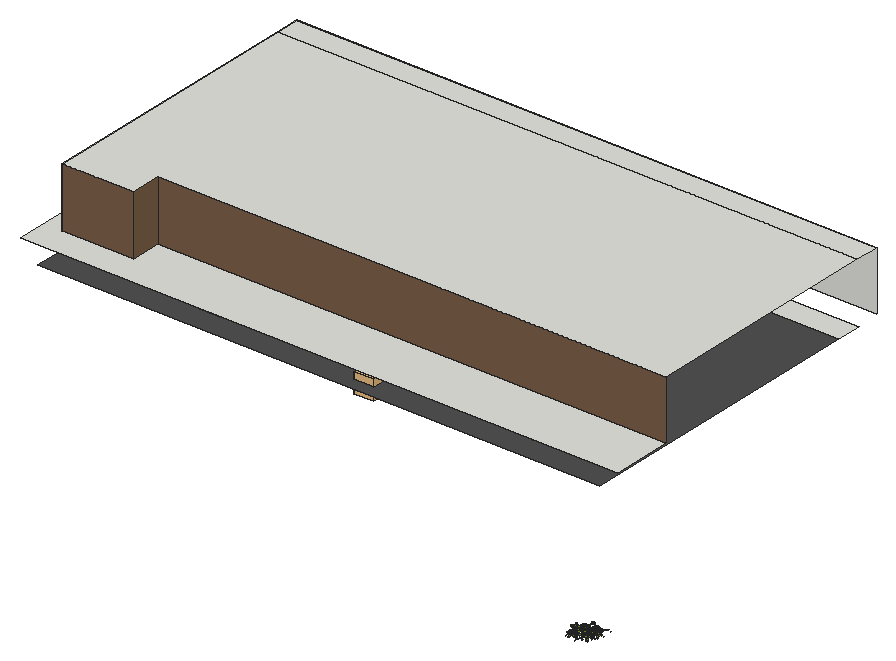
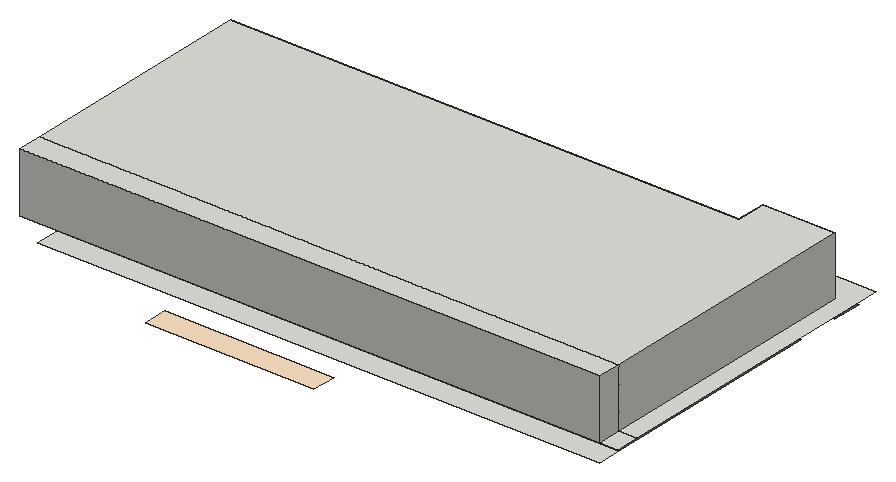
# SketchUp Ruby script. Lengths in inches.
U = 1.inch
M = Sketchup.active_model
def pt(a) = Geom::Point3d.new(a.map { |v| v * U })
def face(e, loops, mat)
  f = e.add_face(loops[0].map { |a| pt(a) })
  loops[1..].each { |l| e.add_face(l.map { |a| pt(a) }).erase! }
  f.material = f.back_material = mat if mat
  f
end
# faces: each face lists its corners as indices into pts; further lists are holes
def faces(e, pts, list, mat = nil) = list.each { |f| face(e, (f[0].is_a?(Array) ? f : [f]).map { |l| l.map { |i| pts[i] } }, mat) }
# xy, xz, yz: faces in a plane at the given z, y or x. An outline is a flat list of corners, or four numbers for a rectangle; further outlines are holes
def ring(l) = l.size == 4 ? [[l[0], l[1]], [l[2], l[1]], [l[2], l[3]], [l[0], l[3]]] : l.each_slice(2).to_a
def flat(e, list, mat, &to3) = list.each { |f| face(e, (f[0].is_a?(Array) ? f : [f]).map { |l| ring(l).map { |u, v| to3.(u, v) } }, mat) }
def xy(e, z, list, mat = nil) = flat(e, list, mat) { |x, y| [x, y, z] }
def xz(e, y, list, mat = nil) = flat(e, list, mat) { |x, z| [x, y, z] }
def yz(e, x, list, mat = nil) = flat(e, list, mat) { |y, z| [x, y, z] }
def lines(e, pts, list) = list.each { |a, b| e.add_line(pt(pts[a]), pt(pts[b])) }
# prism: a flat outline (further loops are holes) pulled along v
def prism(e, loops, v, mat = nil)
  f = face(e, loops, mat); d = Geom::Vector3d.new(v.map { |x| x * U })
  f.pushpull(f.normal.samedirection?(d) ? d.length : -d.length)
end
def box(e, o, s, mat = nil) = prism(e, [[o, [o[0] + s[0], o[1], o[2]], [o[0] + s[0], o[1] + s[1], o[2]], [o[0], o[1] + s[1], o[2]]]], [0, 0, s[2]], mat)
def at(x, y, z, deg = 0) = Geom::Transformation.translation(pt([x, y, z])) * Geom::Transformation.rotation(ORIGIN, Z_AXIS, deg.degrees)
def axes(o, x, y, z) = Geom::Transformation.new([*x, 0, *y, 0, *z, 0, *pt(o).to_a, 1])
def part(name) = M.definitions.add(name)
# library, detail: a bought-in or finely detailed component or shape, given as its bounding box
def library(name, o, s) = part(name).tap { |d| box(d.entities, o, s) }
def detail(e, o, s) = box(e.add_group.entities, o, s)
def put(e, d, t, mat = nil) = e.add_instance(d, t).tap { |i| i.material = mat if mat }
def group(e, t, mat = nil) = e.add_group.tap { |g| g.transformation = t; g.material = mat if mat }.entities
root = M.entities
M.materials.add("[0012_Bisque]").color = [255, 228, 196]
M.materials.add("[0050_LemonChiffon]").color = [255, 250, 205]
M.materials.add("[0054_LightYellow]").color = [255, 255, 224]
M.materials.add("[0061_OliveDrab]").color = [107, 142, 35]
M.materials.add("[0135_DarkGray]").color = [81, 81, 81]
M.materials.add("[Cladding Siding Tan]").color = [124, 97, 73]
c1 = library("Sphere Light\#1",[-9.875,-9.875,-9.875],[19.75,19.75,19.75])
c2 = library("Sphere Light\#2",[-9.875,-9.875,-9.875],[19.75,19.75,19.75])
c3 = library("Sphere Light",[-9.875,-9.875,-9.875],[19.75,19.75,19.75])
xy(root,667.5,[[304.95,312,474.45,336]],"[0012_Bisque]")
xy(root,702,[[18,312,582,336]])
xy(root,702,[[170.5,36.91,167.95,37.24,165.5625,38.23,163.52,39.8,161.95,41.85,160.96,44.23,160.625,46.78,160.96,49.34,161.95,51.72,163.52,53.77,165.5625,55.34,167.95,56.32,170.5,56.66,173.06,56.32,175.4375,55.34,177.48,53.77,179.05,51.72,180.04,49.34,180.375,46.78,180.04,44.23,179.05,41.85,177.48,39.8,175.4375,38.23,173.06,37.24]],"[0050_LemonChiffon]")
xy(root,702,[[335.0625,36.91,332.51,37.24,330.125,38.23,328.08,39.8,326.51,41.85,325.52,44.23,325.1875,46.78,325.52,49.34,326.51,51.72,328.08,53.77,330.125,55.34,332.51,56.32,335.0625,56.66,337.62,56.32,340,55.34,342.05,53.77,343.62,51.72,344.6,49.34,344.9375,46.78,344.6,44.23,343.62,41.85,342.05,39.8,340,38.23,337.62,37.24],[504.5625,36.91,502.01,37.24,499.625,38.23,497.58,39.8,496.01,41.85,495.02,44.23,494.6875,46.78,495.02,49.34,496.01,51.72,497.58,53.77,499.625,55.34,502.01,56.32,504.5625,56.66,507.12,56.32,509.5,55.34,511.55,53.77,513.12,51.72,514.1,49.34,514.4375,46.78,514.1,44.23,513.12,41.85,511.55,39.8,509.5,38.23,507.12,37.24]],"[0054_LightYellow]")
xy(root,702,[[[18,12,18,42,90,42,90,72,240,72,240,84,18,84,18,312,582,312,582,12],[170.5,36.91,173.06,37.24,175.4375,38.23,177.48,39.8,179.05,41.85,180.04,44.23,180.375,46.78,180.04,49.34,179.05,51.72,177.48,53.77,175.4375,55.34,173.06,56.32,170.5,56.66,167.95,56.32,165.5625,55.34,163.52,53.77,161.95,51.72,160.96,49.34,160.625,46.78,160.96,44.23,161.95,41.85,163.52,39.8,165.5625,38.23,167.95,37.24],[335.0625,36.91,337.62,37.24,340,38.23,342.05,39.8,343.62,41.85,344.6,44.23,344.9375,46.78,344.6,49.34,343.62,51.72,342.05,53.77,340,55.34,337.62,56.32,335.0625,56.66,332.51,56.32,330.125,55.34,328.08,53.77,326.51,51.72,325.52,49.34,325.1875,46.78,325.52,44.23,326.51,41.85,328.08,39.8,330.125,38.23,332.51,37.24],[504.5625,36.91,507.12,37.24,509.5,38.23,511.55,39.8,513.12,41.85,514.1,44.23,514.4375,46.78,514.1,49.34,513.12,51.72,511.55,53.77,509.5,55.34,507.12,56.32,504.5625,56.66,502.01,56.32,499.625,55.34,497.58,53.77,496.01,51.72,495.02,49.34,494.6875,46.78,495.02,44.23,496.01,41.85,497.58,39.8,499.625,38.23,502.01,37.24]]],"[0135_DarkGray]")
xy(root,720,[[0,12,600,12,600,72,90,72,90,42,18,42,18,312,0,312],[0,312,18,336]])
xy(root,780,[[18,42,90,42,90,72,600,72,600,312,18,312],[18,312,600,336]])
xz(root,42,[[18,720,90,780]],"[Cladding Siding Tan]")
xz(root,72,[[90,720,600,780]],"[Cladding Siding Tan]")
xz(root,336,[[18,720,600,780]])
yz(root,18,[[42,720,312,780],[312,720,336,780]])
yz(root,90,[[42,720,72,780]],"[Cladding Siding Tan]")
p = [[564.29,5.1875,560.78],[564.12,5.33,560.78],[562.93,3.75,559.05],[561.79,8.16,559.04],[561.59,8.49,559.04],[560.2,7.625,561.09],
  [560.36,7.35,561.09],[573.22,17.34,559.04],[573.47,17.11,559.04],[574.44,18.17,561.23],[574.25,18.36,561.23],[559.27,9.62,561],
  [559.09,9.66,561],[558.8,7.87,559.1],[566.09,10.13,560.93],[565.87,10.1,560.93],[566.23,8.25,559.11],[554.1,19.08,560.81],
  [554.27,19.22,560.81],[552.92,20.64,559.06],[549.52,22.11,560.79],[549.58,22.3125,560.79],[547.63,22.78,559.09],[567.24,8.58,559.22],
  [566.95,8.82,559.22],[565.76,7.36,561.05],[566,7.16,561.05],[570.125,9.75,559.22],[569.9,9.45,559.22],[570.88,8.76,561.55],
  [571.0625,9.01,561.55],[556.11,23.33,561.13],[555.97,23.45,561.13],[554.89,22.05,559.1875],[571.21,27.76,559.17],[571.48,27.51,559.17],
  [572.73,28.93,560.99],[572.51,29.13,560.99],[557.76,29.01,559.24],[557.83,28.63,559.24],[559.08,28.89,561.53],[559.03,29.2,561.53],
  [559.84,9.14,559.32],[559.55,9.32,559.32],[558.6875,7.88,561.34],[558.92,7.74,561.34],[557.04,9.63,559.34],[556.76,9.86,559.34],
  [555.7,8.53,561.34],[555.93,8.34,561.34],[559.59,9.21,559.33],[559.21,9.31,559.33],[559.125,8.81,561.9],[559.43,8.74,561.9],
  [559.85,9.31,559.35],[560.18,9.4,559.35],[559.76,10.89,561.46],[559.48,10.82,561.46],[569.45,10.46,559.34],[569.75,10.28,559.34],
  [570.17,11.08,561.81],[569.93,11.22,561.81],[572.375,13.1875,559.3],[572.11,13.4,559.3],[571.79,12.94,561.86],[572.01,12.77,561.86],
  [553.34,16.17,559.34],[553.05,15.98,559.34],[553.48,15.37,561.85],[553.72,15.52,561.85],[557.53,17.27,561.0625],[557.37,17.39,561.0625],
  [556.28,15.83,559.26],[572.23,16.52,559.35],[572.37,16.18,559.35],[572.5,16.27,561.97],[572.39,16.54,561.97],[574.33,18.23,561.04],
  [574.2,18.04,561.04],[575.89,17.03,559.29],[550.33,19.14,560.92],[550.49,19.27,560.92],[549.12,20.79,559.27],[552.93,20.14,559.31],
  [553.14,20.4,559.31],[552,21.29,561.49],[551.82,21.08,561.49],[553.2,21.02,559.32],[552.94,21.24,559.32],[552.26,20.38,561.7],
  [552.47,20.2,561.7],[573.49,22.4,561],[573.5625,22.19,561],[575.375,22.93,559.25],[572.35,24.65,559.26],[572.42,25.02,559.26],
  [572.06,25.05,561.86],[572,24.75,561.86],[571.86,25.09,559.32],[571.74,25.43,559.32],[571.25,25.22,561.89],[571.35,24.95,561.89],
  [560.84,25.625,561.04],[561.05,25.72,561.04],[560.1,27.49,559.34],[563.4,28.35,559.34],[563.71,28.59,559.34],[563.04,29.37,561.76],
  [562.79,29.17,561.76],[569.4375,29.21,560.97],[569.57,29.07,560.97],[570.95,30.55,559.29],[555.47,10.89,559.35],[555.15,10.82,559.35],
  [555.51,9.39,561.52],[555.77,9.44,561.52],[569.34,11.16,559.43],[569.52,10.83,559.43],[570.57,11.45,561.76],[570.43,11.72,561.76],
  [554.07,13.21,559.4375],[554.42,13.3,559.4375],[554.05,14.52,561.73],[553.77,14.44,561.73],[553.33,14.41,559.36],[553.51,14.7,559.36],
  [552.36,15.38,561.62],[552.21,15.14,561.62],[553.15,15.55,559.36],[553.4375,15.78,559.36],[552.18,17.27,561.11],[551.95,17.08,561.11],
  [570.58,22.38,560.95],[570.46,22.21,560.95],[572.24,21.06,559.4],[553.25,21.39,559.39],[553.62,21.33,559.39],[553.85,23.12,561.29],
  [553.55,23.17,561.29],[558.83,28,559.41],[559.1875,28.09,559.41],[558.78,29.74,561.41],[558.49,29.67,561.41],[574.3125,31.04,560.96],
  [574.47,30.89,560.96],[575.84,32.54,559.4375],[554.22,6.35,561.21],[554.0625,6.49,561.21],[552.86,4.88,559.51],[559.92,10.61,559.5],
  [560.09,10.89,559.5],[558.37,11.94,561.17],[558.23,11.72,561.17],[568.48,11.27,559.5],[568.37,11.64,559.5],[567.33,11.29,561.89],
  [567.42,10.99,561.89],[556.67,11.94,559.5],[556.45,12.19,559.5],[555.53,11.35,561.81],[555.71,11.14,561.81],[555.46,12.43,559.49],
  [555.11,12.39,559.49],[555.25,11.41,561.93],[555.54,11.44,561.93],[561.33,11.84,559.5],[561.36,12.23,559.5],[560.08,12.3,561.79],
  [560.06,11.98,561.79],[565.09,12.41,559.5],[565.22,12.04,559.5],[566.55,12.54,561.71],[566.44,12.85,561.71],[560.24,13.86,559.5],
  [559.93,13.93,559.5],[559.59,12.2,561.45],[559.85,12.14,561.45],[565.57,14.58,559.5],[565.19,14.53,559.5],[565.48,12.67,561.33],
  [565.78,12.71,561.33],[568.1875,12.74,559.5],[568.52,12.67,559.5],[568.82,14.23,561.59],[568.55,14.29,561.59],[563.4,13.59,559.5],
  [563.23,13.25,559.5],[564,12.91,561.99],[564.14,13.1875,561.99],[558.86,13.37,561.3],[559.06,13.42,561.3],[558.46,15.28,559.54],
  [554.43,13.97,559.5],[554.75,13.8,559.5],[555.3,14.92,561.8125],[555.04,15.05,561.8125],[567.01,15.08,559.5],[566.73,14.89,559.5],
  [567.44,13.9,561.82],[567.67,14.06,561.82],[556.66,15.29,559.5],[556.42,15.56,559.5],[555.2,14.37,561.5],[555.4,14.15,561.5],
  [563.9375,14.78,559.5],[563.6875,14.99,559.5],[563.26,14.45,562.03],[563.46,14.27,562.03],[565.76,15.46,559.5],[565.6875,15.15,559.5],
  [566.84,14.92,561.85],[566.89,15.17,561.85],[561.3,15.32,559.5],[561.48,15,559.5],[562.44,15.57,561.875],[562.29,15.84,561.875],
  [557.04,15.51,559.5],[557.33,15.75,559.5],[555.99,17.27,561.17],[555.75,17.07,561.17],[562.11,18.08,559.5],[561.77,18,559.5],
  [562.26,16.15,561.3],[562.53,16.22,561.3],[564.8,16.47,559.5],[564.95,16.11,559.5],[565.97,16.61,561.87],[565.84,16.9,561.87],
  [563.02,16.39,559.5],[563.24,16.64,559.5],[561.9375,17.76,561.49],[561.76,17.55,561.49],[567.9,18.09,559.5],[567.54,18.08,559.5],
  [567.61,16.95,561.87],[567.9,16.96,561.87],[561.3,18.26,559.5],[560.99,18.06,559.5],[561.4,17.51,562.04],[561.65,17.68,562.04],
  [560.57,17.86,559.5],[560.51,18.21,559.5],[559.22,17.93,561.77],[559.28,17.65,561.77],[570.41,18.94,559.5],[570.08,18.9,559.5],
  [570.24,18.01,561.97],[570.51,18.05,561.97],[560.66,18.375,559.5],[560.93,18.1875,559.5],[561.875,19.61,561.5],[561.66,19.76,561.5],
  [563.25,19.7,559.5],[562.95,19.9,559.5],[562.25,18.8125,561.78],[562.49,18.65,561.78],[568.65,19.21,559.5],[568.49,19.48,559.5],
  [567.62,18.91,561.91],[567.76,18.69,561.91],[556.41,19.01,559.5],[556.73,18.89,559.5],[557.18,20.17,561.75],[556.92,20.27,561.75],
  [562.67,19.18,559.5],[563,19.27,559.5],[562.6,20.65,561.7],[562.34,20.58,561.7],[560.3,20.71,559.5],[560.03,20.92,559.5],
  [558.9375,19.47,561.4],[559.16,19.3,561.4],[570.66,20.8125,559.5],[570.4375,20.49,559.5],[572.02,19.46,561.33],[572.2,19.73,561.33],
  [566.75,20.12,559.5],[567.07,20.33,559.5],[566.49,21.15,561.93],[566.22,20.98,561.93],[569.2,21,559.5],[569.32,20.64,559.5],
  [571.11,21.3,561.31],[571.01,21.59,561.31],[553.97,20.71,559.5],[554.07,21.05,559.5],[552.08,21.61,561.12],[552,21.33,561.12],
  [566.52,20.66,559.5],[566.9,20.76,559.5],[566.43,22.39,561.5],[566.125,22.31,561.5],[558.6,22.79,559.5],[558.22,22.68,559.5],
  [558.7,21.09,561.53],[559.01,21.17,561.53],[558.51,21.09,559.5],[558.83,21.08,559.5],[558.84,21.78,562.03],[558.58,21.79,562.03],
  [561.125,21.4375,559.5],[561.39,21.15,559.5],[562.82,22.51,561.23],[562.6,22.75,561.23],[559.14,21.95,559.5],[558.96,21.67,559.5],
  [559.66,21.27,562],[559.8,21.5,562],[565.32,23.03,559.5],[565,23.17,559.5],[564.34,21.56,561.47],[564.6,21.45,561.47],
  [562.68,21.48,559.5],[563.04,21.65,559.5],[562.19,23.375,561.29],[561.9,23.24,561.29],[565.33,22.04,559.5],[565.26,22.37,559.5],
  [563.49,21.98,561.4],[563.55,21.71,561.4],[561.8,22.32,559.5],[561.61,22.6,559.5],[560.88,22.05,561.96],[561.04,21.82,561.96],
  [559.53,21.875,559.5],[559.84,22.04,559.5],[559.3,23,561.88],[559.05,22.87,561.88],[554.89,22.22,559.5],[555.25,22.23,559.5],
  [555.15,24.0625,561.38],[554.86,24.05,561.38],[565.91,22.61,559.5],[565.98,22.28,559.5],[566.875,22.52,561.96],[566.8125,22.78,561.96],
  [558.59,23.02,559.5],[558.43,23.3,559.5],[557.4375,22.69,561.85],[557.56,22.47,561.85],[565.38,23.52,559.5],[565.2,23.21,559.5],
  [566.52,22.48,561.65],[566.67,22.73,561.65],[569.3,23.05,559.5],[569.58,23.25,559.5],[568.69,24.39,561.69],[568.47,24.22,561.69],
  [563.03,24.21,559.5],[562.84,24.47,559.5],[561.56,23.47,561.5625],[561.71,23.26,561.5625],[566.83,25.18,559.5],[566.62,24.89,559.5],
  [568.31,23.71,561.12],[568.48,23.95,561.12],[560.31,24.77,559.5],[560.04,24.98,559.5],[559.31,23.97,561.81],[559.52,23.8,561.81],
  [564.5625,24.49,561.07],[564.71,24.32,561.07],[566.17,25.8125,559.47],[562.52,26.07,559.5],[562.29,25.76,559.5],[563.58,24.85,561.6],
  [563.76,25.1,561.6],[555.8125,26.02,559.5],[555.64,25.73,559.5],[557.01,24.97,561.61],[557.15,25.21,561.61],[558.875,26.46,559.5],
  [558.63,26.67,559.5],[557.62,25.44,561.59],[557.82,25.27,561.59],[566.09,26.05,559.5],[566.32,25.82,559.5],[567.72,27.22,561.22],
  [567.53,27.41,561.22],[565.77,27.27,559.5],[565.53,27.54,559.5],[564.14,26.22,561.3],[564.34,26.01,561.3],[563.12,13.66,561.1875],
  [562.92,13.61,561.1875],[563.52,11.61,559.6],[556.03,13.15,561.07],[556.13,13.3125,561.07],[554.27,14.375,559.56],[560.97,21.23,561.24],
  [560.93,21.41,561.24],[558.97,20.92,559.5625],[565.83,23.49,561.42],[565.7,23.3125,561.42],[567.32,22.24,559.66],[562.375,24.27,561.22],
  [562.24,24.42,561.22],[560.75,22.92,559.66],[559.59,21.72,561.49],[559.48,21.87,561.49],[557.92,20.59,559.81],[557.88,22.71,561.62],
  [558.0625,22.64,561.62],[558.65,24.47,559.83],[565.5,24.86,561.43],[565.72,24.91,561.43],[565.09,26.86,559.77],[554.81,26.68,561.33],
  [555.01,26.69,561.33],[554.84,28.78,559.76],[569.13,16.85,561.61],[569.32,16.81,561.61],[569.65,18.85,560],[558.1,6.06,561.4],
  [557.98,6.25,561.4],[556.1,5,560.0625],[553.98,25.75,561.47],[554.2,25.72,561.47],[554.42,27.94,560.09],[557.5,5.54,561.6],
  [557.34,5.65,561.6],[556.23,3.7,560.23],[568.93,13.67,561.89],[569,13.46,561.89],[570.96,14.26,560.33],[566.94,26.35,561.87],
  [567.1,26.47,561.87],[565.77,28.12,560.32],[563.52,19.0625,561.7],[563.34,19.14,561.7],[562.54,17.04,560.35],[557.95,32.22,561.72],
  [558.16,32.27,561.72],[557.55,34.47,560.43],[556.31,6.91,561.9],[556.13,6.86,561.9],[556.72,4.69,560.54],[559.83,19.31,561.82],
  [559.96,19.45,561.82],[558.18,20.9,560.55],[576.0625,20.19,561.73],[576.2,20.06,561.73],[577.72,21.78,560.46],[563.18,21.88,561.79],
  [563.33,21.77,561.79],[564.55,23.6875,560.47],[553.47,12.41,561.84],[553.33,12.5625,561.84],[551.72,10.91,560.58],[559.65,18.66,561.93],
  [559.43,18.6,561.93],[560.15,16.39,560.7],[555.29,21.21,562.23],[555.2,21.37,562.23],[553.375,20.22,560.73],[557.9,25.19,562.35],
  [558.08,25.28,562.35],[556.98,27.18,560.9],[572.69,12.91,562.33],[572.79,12.72,562.33],[574.74,13.91,561.02],[549.87,22.72,562.11],
  [549.99,22.87,562.11],[548.09,24.29,560.97],[561.73,23.07,562.24],[561.92,23.125,562.24],[561.23,25.35,561.02],[556.75,17.22,562.35],
  [556.71,17.42,562.35],[554.47,16.9,561.09],[559.35,23.9,562.17],[559.25,23.73,562.17],[561.36,22.625,561.05],[568.85,21.41,562.29],
  [568.74,21.23,562.29],[570.87,20.12,561.23],[569.31,23.31,562.59],[569.35,23.12,562.59],[571.5,23.7,561.2],[561.27,31.17,562.51],
  [561.45,31.3125,562.51],[559.92,33.05,561.27],[553.16,16.875,562.51],[553.36,16.93,562.51],[552.64,19.21,561.42],[557.96,21.83,562.56],
  [557.8,21.95,562.56],[556.43,20.01,561.43],[561.48,29.6,562.37],[561.52,29.38,562.37],[563.89,29.93,561.37],[569.06,11.97,562.61],
  [568.89,11.85,562.61],[570.32,9.94,561.52],[571.2,13.33,562.71],[571.37,13.23,562.71],[572.46,15.31,561.53],[565.61,17.42,562.71],
  [565.51,17.57,562.71],[563.57,16.27,561.51],[572.83,7.35,562.6],[572.96,7.53,562.6],[550.27,16.625,562.6],[550.17,16.46,562.6],
  [564.48,17.01,562.73],[564.58,16.82,562.73],[566.62,18.08,561.64],[550.75,18.55,562.82],[550.9,18.43,562.82],[574.9,5.94,561.79],
  [553.7,9.71,562.75],[553.83,9.57,562.75],[557.67,12.45,562.82],[557.66,12.23,562.82],[567.93,14.5,562.78],[567.73,14.49,562.78],
  [567.91,12.08,561.76],[569.18,14.43,562.92],[569.22,14.61,562.92],[556.375,17.06,562.88],[556.19,17.16,562.88],[548.09,17.86,561.82],
  [560.9,16.77,562.73],[561.07,16.66,562.73],[558.75,24.22,563.03],[558.9375,24.21,563.03],[558.97,26.54,561.83],[558.85,7.51,564.16],
  [559.0625,7.45,564.16],[551.9,8.02,561.85],[555.54,9.21,563.33],[555.75,9.23,563.33],[565.04,10.55,562.9375],[565.1,10.34,562.9375],
  [570.47,11.21,563.33],[570.625,11.09,563.33],[554.66,13.61,563.41],[554.83,13.72,563.41],[559.58,14.66,561.89],[568.08,17.6,563.08],
  [567.98,17.81,563.08],[565.24,22.95,563.37],[565.05,22.83,563.37],[569.48,24.5625,563.71],[569.54,24.37,563.71],[570.87,25.22,564.19],
  [570.83,25.01,564.19],[565.91,12.01,563.54],[566.01,12.2,563.54],[561.97,12.88,563.7],[562.11,12.76,563.7],[570.82,15.67,563.04],
  [570.63,15.64,563.04],[571.08,13.26,562.03],[562.42,16.0625,563.97],[562.6,16.18,563.97],[572.95,16.5,564.55],[572.87,16.69,564.55],
  [549.2,16.58,562.04],[561.38,20.24,563.6875],[561.48,20.4,563.6875],[559.125,20.78,563.44],[559.24,20.62,563.44],[562.7,9.73,562.06],
  [555.16,12.55,562.08],[571.65,13.97,562.125],[557.46,19.34,562.15],[570.35,18.75,562.44],[569.01,9.19,562.5],[555.94,6.66,562.86],
  [556.14,11.5,562.92],[557.06,19.21,563],[563.71,25.06,562.98],[568.29,10.95,563.17],[560.35,10.85,563.3125],[567.05,23.61,563.375],
  [563.65,18.93,563.5],[563.97,13.95,564.19],[558.36,5.12,565.14],[568.42,25.56,565.1],[574.26,17.14,566.73],[18,312,720],
  [600,312,720]]
faces(root,p,[[0,1,2],[3,4,5,6],[7,8,9,10],[11,12,13],[14,15,16],[17,18,19],[20,21,22],[23,24,25,26],
  [27,28,29,30],[31,32,33],[34,35,36,37],[38,39,40,41],[42,43,44,45],[46,47,48,49],[50,51,52,53],[54,55,56,57],
  [58,59,60,61],[62,63,64,65],[66,67,68,69],[70,71,72],[73,74,75,76],[77,78,79],[80,81,82],[83,84,85,86],
  [87,88,89,90],[91,92,93],[94,95,96,97],[98,99,100,101],[102,103,104],[105,106,107,108],[109,110,111],[112,113,114,115],
  [116,117,118,119],[120,121,122,123],[124,125,126,127],[128,129,130,131],[132,133,134],[135,136,137,138],[139,140,141,142],[143,144,145],
  [146,147,148],[149,150,151,152],[153,154,155,156],[157,158,159,160],[161,162,163,164],[165,166,167,168],[169,170,171,172],[173,174,175,176],
  [177,178,179,180],[181,182,183,184],[185,186,187,188],[189,190,191],[192,193,194,195],[196,197,198,199],[200,201,202,203],[204,205,206,207],
  [208,209,210,211],[212,213,214,215],[216,217,218,219],[220,221,222,223],[224,225,226,227],[228,229,230,231],[232,233,234,235],[236,237,238,239],
  [240,241,242,243],[244,245,246,247],[248,249,250,251],[252,253,254,255],[256,257,258,259],[260,261,262,263],[264,265,266,267],[268,269,270,271],
  [272,273,274,275],[276,277,278,279],[280,281,282,283],[284,285,286,287],[288,289,290,291],[292,293,294,295],[296,297,298,299],[300,301,302,303],
  [304,305,306,307],[308,309,310,311],[312,313,314,315],[316,317,318,319],[320,321,322,323],[324,325,326,327],[328,329,330,331],[332,333,334,335],
  [336,337,338,339],[340,341,342,343],[344,345,346,347],[348,349,350,351],[352,353,354,355],[356,357,358,359],[360,361,362],[363,364,365,366],
  [367,368,369,370],[371,372,373,374],[375,376,377,378],[379,380,381,382],[383,384,385],[386,387,388],[389,390,391],[392,393,394],
  [395,396,397],[398,399,400],[401,402,403],[404,405,406],[407,408,409],[410,411,412],[413,414,415],[416,417,418],
  [419,420,421],[422,423,424],[425,426,427],[428,429,430],[431,432,433],[434,435,436],[437,438,439],[440,441,442],
  [443,444,445],[446,447,448],[449,450,451],[452,453,454],[26,25,1,0],[219,218,18,17],[287,286,21,20],[180,179,15,14],
  [131,130,81,80],[455,456,457],[176,175,12,11],[458,459,460],[275,274,78,77],[283,282,92,91],[355,354,133,132],[461,462,463],
  [464,465,466],[315,314,103,102],[378,377,110,109],[37,36,144,143],[6,5,414,413],[152,151,387,386],[467,468,469],[271,270,71,70],
  [303,302,361,360],[470,471,472],[374,373,32,31],[49,48,147,146],[223,222,384,383],[10,9,441,440],[473,474,475],[319,318,390,389],
  [476,477,478],[382,381,396,395],[45,44,420,419],[57,56,190,189],[138,137,417,416],[331,330,408,407],[479,480,481],[482,483,484],
  [485,486,487],[291,290,405,404],[366,365,393,392],[488,489,490],[142,141,432,431],[115,114,435,434],[491,492,493],[203,202,447,446],
  [494,495,496],[497,498,499],[231,230,438,437],[295,294,450,449],[311,310,429,428],[251,250,444,443],[86,85,462,461],[351,350,399,398],
  [41,40,489,488],[30,29,500,501],[184,183,411,410],[127,126,502,503],[504,505,506],[263,262,402,401],[343,342,474,473],[370,369,471,470],
  [172,171,423,422],[123,122,483,482],[90,89,507,508],[267,266,465,464],[347,346,426,425],[501,500,509],[160,159,510,511],[61,60,495,494],
  [119,118,459,458],[199,198,492,491],[168,167,512,513],[514,515,516],[211,210,517,518],[195,194,519,520],[503,502,521],[255,254,522,523],
  [243,242,468,467],[359,358,486,485],[524,525,526],[108,107,480,479],[53,52,527,528],[511,510,529],[164,163,530,531],[156,155,532,533],
  [65,64,534,535],[69,68,536,537],[235,234,515,514],[523,522,538],[215,214,505,504],[227,226,539,540],[259,258,498,497],[279,278,541,542],
  [339,338,453,452],[327,326,456,455],[101,100,543,544],[97,96,545,546],[188,187,547,548],[207,206,549,550],[551,552,553],[247,246,552,551],
  [239,238,554,555],[76,75,556,557],[508,507,558],[307,306,559,560],[323,322,561,562],[299,298,525,524],[335,334,477,476],[533,532,563],
  [513,512,564],[518,517,565],[520,519,566],[540,539,567],[535,534,568],[531,530,569],[537,536,570],[562,561,571],
  [542,541,572],[548,547,573],[550,549,574],[544,543,575],[560,559,576],[555,554,577],[528,527,578],[546,545,579],
  [557,556,580]],"[0061_OliveDrab]")
lines(root,p,[[581,582]])
put(root,c1,at(334.74,34.67,698.5625))
put(root,c2,at(504.5625,46.78,700.625))
put(root,c3,at(170.5,46.78,702))
